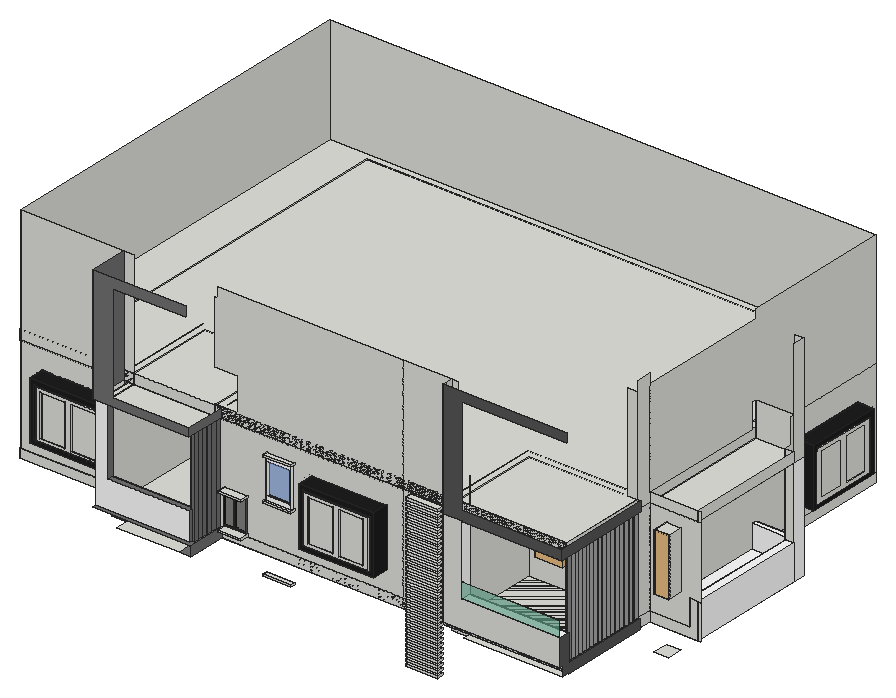
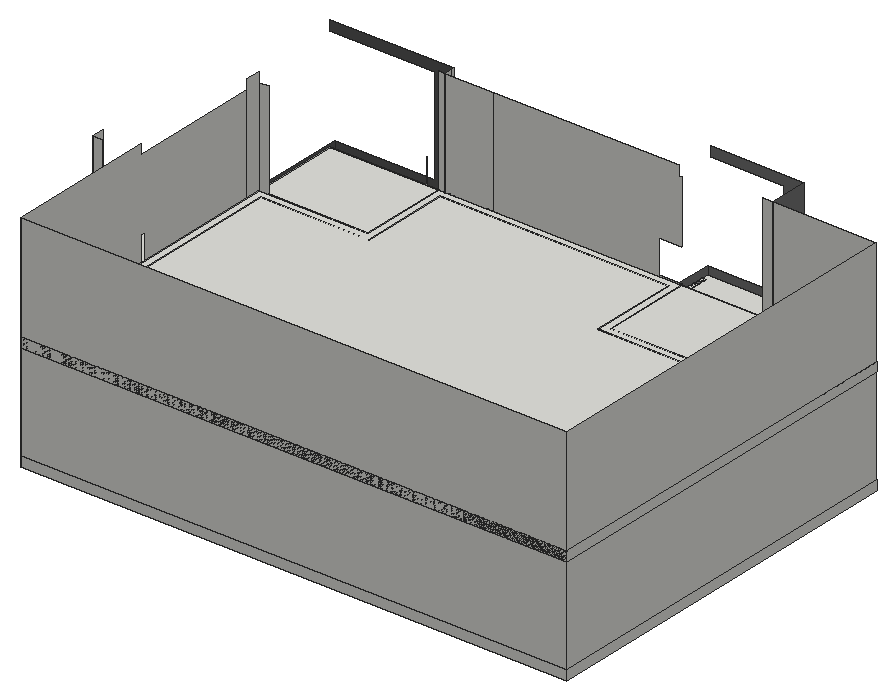
# SketchUp Ruby script. Lengths in inches.
U = 1.inch
M = Sketchup.active_model
def pt(a) = Geom::Point3d.new(a.map { |v| v * U })
def face(e, loops, mat)
  f = e.add_face(loops[0].map { |a| pt(a) })
  loops[1..].each { |l| e.add_face(l.map { |a| pt(a) }).erase! }
  f.material = f.back_material = mat if mat
  f
end
# faces: each face lists its corners as indices into pts; further lists are holes
def faces(e, pts, list, mat = nil) = list.each { |f| face(e, (f[0].is_a?(Array) ? f : [f]).map { |l| l.map { |i| pts[i] } }, mat) }
# xy, xz, yz: faces in a plane at the given z, y or x. An outline is a flat list of corners, or four numbers for a rectangle; further outlines are holes
def ring(l) = l.size == 4 ? [[l[0], l[1]], [l[2], l[1]], [l[2], l[3]], [l[0], l[3]]] : l.each_slice(2).to_a
def flat(e, list, mat, &to3) = list.each { |f| face(e, (f[0].is_a?(Array) ? f : [f]).map { |l| ring(l).map { |u, v| to3.(u, v) } }, mat) }
def xy(e, z, list, mat = nil) = flat(e, list, mat) { |x, y| [x, y, z] }
def xz(e, y, list, mat = nil) = flat(e, list, mat) { |x, z| [x, y, z] }
def yz(e, x, list, mat = nil) = flat(e, list, mat) { |y, z| [x, y, z] }
def lines(e, pts, list) = list.each { |a, b| e.add_line(pt(pts[a]), pt(pts[b])) }
# prism: a flat outline (further loops are holes) pulled along v
def prism(e, loops, v, mat = nil)
  f = face(e, loops, mat); d = Geom::Vector3d.new(v.map { |x| x * U })
  f.pushpull(f.normal.samedirection?(d) ? d.length : -d.length)
end
def box(e, o, s, mat = nil) = prism(e, [[o, [o[0] + s[0], o[1], o[2]], [o[0] + s[0], o[1] + s[1], o[2]], [o[0], o[1] + s[1], o[2]]]], [0, 0, s[2]], mat)
def at(x, y, z, deg = 0) = Geom::Transformation.translation(pt([x, y, z])) * Geom::Transformation.rotation(ORIGIN, Z_AXIS, deg.degrees)
def axes(o, x, y, z) = Geom::Transformation.new([*x, 0, *y, 0, *z, 0, *pt(o).to_a, 1])
def part(name) = M.definitions.add(name)
# library, detail: a bought-in or finely detailed component or shape, given as its bounding box
def library(name, o, s) = part(name).tap { |d| box(d.entities, o, s) }
def detail(e, o, s) = box(e.add_group.entities, o, s)
def put(e, d, t, mat = nil) = e.add_instance(d, t).tap { |i| i.material = mat if mat }
def group(e, t, mat = nil) = e.add_group.tap { |g| g.transformation = t; g.material = mat if mat }.entities
root = M.entities
M.materials.add("Glass_Tinted_Gray").color = [0, 0, 0]
M.materials["Glass_Tinted_Gray"].alpha = 0.125
M.materials.add("MaterialE").color = [182, 131, 172]
M.materials["MaterialE"].alpha = 0.66
M.materials.add("MaterialF").color = [114, 188, 161]
M.materials["MaterialF"].alpha = 0.66
M.materials.add("[0135_DarkGray]").color = [81, 81, 81]
M.materials.add("[Color M00]").color = [255, 255, 255]
M.materials.add("[Color M03]").color = [170, 170, 170]
M.materials.add("[Color M04]").color = [142, 142, 142]
M.materials.add("[Color M05]").color = [114, 114, 114]
M.materials.add("[Color M06]").color = [86, 86, 86]
M.materials.add("[Color M08]").color = [30, 30, 30]
M.materials.add("[Color_000]").color = [255, 255, 255]
M.materials.add("[Mirror 02]1").color = [229, 229, 229]
M.materials.add("[Terrazzo Light Blue]").color = [196, 214, 227]
M.materials.add("[Translucent Glass Blue]").color = [100, 149, 237]
M.materials["[Translucent Glass Blue]"].alpha = 0.5
c1 = part("Group\#4")
box(c1.entities,[0,0,0],[39.5625,8.625,2.78])
c2 = part("Group\#73")
box(c2.entities,[0,0,0],[34.1875,2.25,6.125])
c3 = part("Group\#3")
box(c3.entities,[3,0,0],[2.8125,4.1875,120.875])
c4 = part("Group\#76")
box(c4.entities,[0,0,0],[4.8125,4.8125,120],"[Color M05]")
c5 = part("Group\#75")
box(c5.entities,[0,-10.375,0],[28.375,10.375,2.5])
c6 = part("PENTEK_RP Fineline 50S_Sliding_DoorCase_E1")
box(c6.entities,[0,0,0],[1.51,3.66,99.27],"[0135_DarkGray]")
c7 = part("PENTEK_RP Fineline 50S_SlidingDooe_Case_E2")
box(c7.entities,[0,0,0],[96.25,3.66,1.51],"[0135_DarkGray]")
c8 = part("pentek_RP Fineline 50S_SlidingDoor_Case")
put(c8.entities,c6,at(97.76,0,0))
put(c8.entities,c7,at(1.51,0,0))
put(c8.entities,c6,at(0,0,0))
put(c8.entities,c7,at(1.51,0,97.76))
c9 = part("PENTEK_RP Fineline 50S_SlidingDoor_GlazingBead_2")
box(c9.entities,[0,0,0],[0.56,0.59,94.39],"[0135_DarkGray]")
c10 = part("PENTEK_RP Fineline 50S_SlidingDoor_Glass")
box(c10.entities,[0,0,0],[46.58,0.16,94.39],"Glass_Tinted_Gray")
c11 = part("PENTEK_RP Fineline 50S_SlidingDoor_GlazingBead")
box(c11.entities,[0,0,0],[45.47,0.59,0.56],"[0135_DarkGray]")
c12 = part("PENTEK_RP Fineline 50S_SlidingDoor_Leaf_E1")
xy(c12.entities,0,[[0,0,0.93,1.97],[0.93,1.57,1.49,1.97]],"[0135_DarkGray]")
xy(c12.entities,96.25,[[0,0,0.93,0,0.93,1.57,1.49,1.57,1.49,1.97,0,1.97]],"[0135_DarkGray]")
xz(c12.entities,0,[[0,0,0.93,96.25]],"[0135_DarkGray]")
xz(c12.entities,1.57,[[0.93,0,1.49,95.32],[0.93,95.32,1.49,96.25]],"[0135_DarkGray]")
xz(c12.entities,1.97,[[0,0,1.49,96.25]],"[0135_DarkGray]")
yz(c12.entities,0,[[0,0,1.97,96.25]],"[0135_DarkGray]")
yz(c12.entities,0.93,[[0,0,1.57,0.93],[0,0.93,1.57,95.32],[0,95.32,1.57,96.25]],"[0135_DarkGray]")
yz(c12.entities,1.49,[[1.57,0,1.97,95.32],[1.57,95.32,1.97,96.25]],"[0135_DarkGray]")
c13 = part("PENTEK_RP Fineline 50S_SlidingDoor_Leaf_E2")
xy(c13.entities,0,[[0,0,0,1.57,0.56,1.57,0.56,1.97,46.02,1.97,46.02,1.57,46.58,1.57,46.58,0]],"[0135_DarkGray]")
xy(c13.entities,0.93,[[0,0,46.58,1.57]],"[0135_DarkGray]")
xy(c13.entities,1.49,[[0.56,1.57,46.02,1.97]],"[0135_DarkGray]")
xz(c13.entities,0,[[0,0,46.58,0.93]],"[0135_DarkGray]")
xz(c13.entities,1.57,[[0,0,0.56,0.93],[46.02,0,46.58,0.93],[0.56,0.93,46.02,1.49]],"[0135_DarkGray]")
xz(c13.entities,1.97,[[0.56,0,46.02,1.49]],"[0135_DarkGray]")
yz(c13.entities,0,[[0,0,1.57,0.93]],"[0135_DarkGray]")
yz(c13.entities,0.56,[[1.57,0,1.97,0.93],[1.57,0.93,1.97,1.49]],"[0135_DarkGray]")
yz(c13.entities,46.02,[[1.57,0,1.97,0.93],[1.57,0.93,1.97,1.49]],"[0135_DarkGray]")
yz(c13.entities,46.58,[[0,0,1.57,0.93]],"[0135_DarkGray]")
c14 = part("PENTEK_RP Fineline S_SlidingDoor_Leaf1")
put(c14.entities,c9,at(0.93,0,0.93))
put(c14.entities,c9,at(46.96,0,0.93))
put(c14.entities,c10,at(1.49,1.42,0.93))
put(c14.entities,c11,at(1.49,0,0.93))
put(c14.entities,c10,at(1.49,0.59,0.93),"[Terrazzo Light Blue]")
put(c14.entities,c12,at(0,0,0))
put(c14.entities,c12,axes([48.44,0,0],[-1,0,0],[0,1,0],[0,0,1]))
put(c14.entities,c13,axes([0.93,0,96.25],[1,0,0],[0,1,0],[0,0,-1]))
put(c14.entities,c13,at(0.93,0,0))
put(c14.entities,c11,at(1.49,0,94.77))
c15 = part("PENTEK_RP Fineline 50S_SlidingDoor_Leaf2")
put(c15.entities,c10,at(1.49,1.42,0.93))
put(c15.entities,c11,at(1.49,0,94.77))
put(c15.entities,c9,at(46.96,0,0.93))
put(c15.entities,c10,at(1.49,0.59,0.93),"[Mirror 02]1")
put(c15.entities,c9,at(0.93,0,0.93))
put(c15.entities,c12,at(0,0,0))
put(c15.entities,c12,axes([48.44,0,0],[-1,0,0],[0,1,0],[0,0,1]))
put(c15.entities,c11,at(1.49,0,0.93))
put(c15.entities,c13,axes([0.93,0,96.25],[1,0,0],[0,1,0],[0,0,-1]))
put(c15.entities,c13,at(0.93,0,0))
c16 = part("PENTEK - Slimmest Steel Sliding Door / Window\#1")
put(c16.entities,c8,at(0,-1.88,-0.09))
put(c16.entities,c14,at(1.51,-2.27,1.42))
put(c16.entities,c15,at(49.32,-0.3,1.42))
c17 = library("Single door",[0,0,0],[7.5,39.86,83.92])
c18 = part("Window")
xy(c18.entities,31.72,[[-0.78,88.6,2.72,128.1]])
xy(c18.entities,34.95,[[-0.78,91.53,0.84,106.59],[0.84,91.53,1.05,97.58],[1.05,91.53,1.42,106.59],[1.42,91.53,2.72,106.59],[0.84,97.58,1.05,98.18],
  [0.84,98.18,1.05,106.59]])
xy(c18.entities,35.27,[[-0.78,110.09,0.97,125.14],[1.05,110.09,2.72,125.14]])
xy(c18.entities,58.35,[[2.72,108.74,3.8,109.74]])
xy(c18.entities,77.8125,[[-0.78,110.09,2.72,125.14],[0.97,110.09,1.05,125.14]])
xy(c18.entities,77.93,[[-0.78,91.53,0.84,106.59],[1.05,91.53,1.42,106.59],[1.42,91.53,2.72,106.59]])
xy(c18.entities,80.72,[[-0.78,88.6,2.72,128.1]])
xz(c18.entities,88.6,[[-0.78,31.72,2.72,80.72]])
xz(c18.entities,91.53,[[-0.78,34.95,0.84,77.93],[1.05,34.95,1.42,77.93],[1.42,34.95,2.72,77.93]])
xz(c18.entities,106.59,[[-0.78,34.95,0.84,77.93],[0.84,34.95,1.05,77.93],[0.84,34.95,2.72,77.93]])
xz(c18.entities,108.74,[[3.8,54.35,4.22,54.6,4.22,59.47,2.72,59.97,2.72,58.35,3.8,58.35]])
xz(c18.entities,109.74,[[3.8,54.35,3.8,58.35,2.72,58.35,2.72,59.97,4.22,59.47,4.22,54.6]])
xz(c18.entities,110.09,[[-0.78,35.27,0.97,77.8125],[1.05,35.27,2.72,77.8125]])
xz(c18.entities,125.14,[[-0.78,35.27,0.97,77.8125],[0.97,35.27,1.05,80.72],[1.05,35.27,2.72,77.8125]])
xz(c18.entities,128.1,[[-0.78,31.72,2.72,80.72]])
yz(c18.entities,-0.78,[[[88.6,31.72,128.1,80.72],[91.53,34.95,106.59,77.93],[110.09,35.27,125.14,77.8125]]])
yz(c18.entities,0.84,[[91.53,34.95,106.59,77.93]])
yz(c18.entities,0.97,[[110.09,35.27,125.14,77.8125]])
yz(c18.entities,1.05,[[91.53,34.95,106.59,77.93],[110.09,35.27,125.14,77.8125]])
yz(c18.entities,1.42,[[91.53,34.95,106.59,77.93]])
yz(c18.entities,2.72,[[[88.6,31.72,108.35,80.72],[91.53,34.95,106.59,77.93]],[[108.35,31.72,128.1,80.72],[110.09,35.27,125.14,77.8125],[108.74,58.35,109.74,59.97]]])
yz(c18.entities,3.8,[[108.74,54.35,109.74,58.35]])
yz(c18.entities,4.22,[[108.74,54.6,109.74,59.47]])
p = [[4.22,108.74,54.6],[3.8,108.74,54.35],[3.8,109.74,54.35],[4.22,109.74,54.6],[2.72,109.74,59.97],[2.72,108.74,59.97],
  [4.22,108.74,59.47],[4.22,109.74,59.47],[-0.78,86.4,89.94],[-0.78,86.44,89.94],[15.22,130.69,89.94],[15.22,130.65,89.94],
  [-0.78,86.44,28.19],[-0.78,86.4,28.19],[7.72,130.69,89.94],[7.72,130.65,89.94]]
faces(c18.entities,p,[[0,1,2,3],[4,5,6,7]])
lines(c18.entities,p,[[8,9],[10,11],[12,13],[14,15]])
c19 = part("Group\#5")
xy(c19.entities,0,[[[0,0,93.5,72.0625],[5.4,5.4,88.1,66.66]],[5.4,5.4,88.1,66.66]])
xy(c19.entities,20.1875,[[[0,0,93.5,72.0625],[5.4,5.4,88.1,66.66]]])
xz(c19.entities,0,[[0,0,93.5,20.1875]])
xz(c19.entities,5.4,[[5.4,0,88.1,20.1875]])
xz(c19.entities,66.66,[[5.4,0,88.1,20.1875]])
xz(c19.entities,72.0625,[[0,0,93.5,20.1875]])
yz(c19.entities,0,[[0,0,72.0625,20.1875]])
yz(c19.entities,5.4,[[5.4,0,66.66,20.1875]])
yz(c19.entities,88.1,[[5.4,0,66.66,20.1875]])
yz(c19.entities,93.5,[[0,0,72.0625,20.1875]])
c20 = library("Sliding Window",[0,0,0],[35.43,4.93,59.06])
c21 = part("glassE")
xy(c21.entities,0,[[0,0,37.99,0.79]],"MaterialE")
xy(c21.entities,38.27,[[0,0,37.99,0.79]],"MaterialE")
xz(c21.entities,0,[[0,0,37.99,38.27]],"MaterialF")
yz(c21.entities,0,[[0,0,0.79,38.27]],"MaterialE")
yz(c21.entities,37.99,[[0,0,0.79,38.27]],"MaterialE")
c22 = library("grille P1",[0,0,0],[0.79,28.9,72.83])
c23 = part("bod vindu")
g1 = group(c23.entities,at(0,-46.85,0),"[Translucent Glass Blue]")
yz(g1,0.94,[[2.36,2.36,44.49,19.65]],"[Translucent Glass Blue]")
p = [[0.55,44.49,2.36],[0.94,44.49,2.36],[0.55,2.36,19.65],[0.94,2.36,19.65]]
lines(g1,p,[[0,1],[2,3]])
g2 = group(g1,at(0,46.85,0,-90),"[Color_000]")
xy(g2,0,[[0,0,46.85,3.9375]])
xy(g2,1.57,[[1.57,0,45.28,0.55]])
xy(g2,2.36,[[2.36,0.55,44.49,3.9375]])
xy(g2,19.65,[[2.36,0.55,4.29,3.9375],[4.29,0.55,44.49,3.9375]])
xy(g2,20.43,[[1.57,0,45.28,0.55]])
xy(g2,22.01,[[0,0,46.85,3.9375]])
xz(g2,0,[[[0,0,46.85,22.01],[1.57,1.57,45.28,20.43]]])
xz(g2,0.55,[[1.57,1.57,45.28,2.36],[1.57,2.36,2.36,2.36,2.36,19.65,44.49,19.65,44.49,2.36,45.28,2.36,45.28,20.43,1.57,20.43]])
xz(g2,3.9375,[[[0,0,46.85,22.01],[2.36,2.36,44.49,19.65]]])
yz(g2,0,[[0,0,3.9375,22.01]])
yz(g2,1.57,[[0,1.57,0.55,2.36,0.55,20.43,0,20.43]])
yz(g2,2.36,[[0.55,2.36,3.9375,19.65]])
yz(g2,44.49,[[0.55,2.36,3.9375,19.65]])
yz(g2,45.28,[[0,1.57,0,20.43,0.55,20.43,0.55,2.36]])
yz(g2,46.85,[[0,0,3.9375,22.01]])
p = [[45.28,0,1.57],[1.57,0,1.57],[1.57,0.55,2.36],[2.36,0.55,2.36],[44.49,0.55,2.36],[45.28,0.55,2.36]]
faces(g2,p,[[0,1,2,3,4,5]])
xy(root,233.98,[[848.78,313.75,867.09,332.62]])
xy(root,252,[[308.96,155.5,308.96,170.3125,291.14,170.3125,291.14,203.9375,386.69,203.9375,386.69,155.5],[386.69,170.3125,392.02,203.9375],[[150.47,203.9375,291.32,203.9375,291.32,313.75,392.02,313.75,392.02,203.9375,693.39,203.9375,693.39,313.75,827.97,313.75,827.97,683.9375,150.47,683.9375],[203.47,212.9375,203.47,674.9375,818.97,674.9375,818.97,322.75,684.39,322.75,684.39,212.9375,401.02,212.9375,401.02,322.75,282.32,322.75,282.32,212.9375]],[818.5,203.9375,827.97,313.75],[828.01,203.9375,830.59,313.75]])
xy(root,252,[[827.97,332.62,887.97,496.51]],"[Color M00]")
xy(root,252,[[386.69,155.5,400.83,170.3125],[392.02,170.3125,400.83,203.9375]],"[Color M05]")
xy(root,252.02,[[707.95,194.4375,830.59,203.9375]])
xy(root,264,[[[284.94,166.84,291.32,166.84,291.32,313.75,392.02,313.75,392.02,203.9375,693.39,203.9375,693.39,313.75,827.97,313.75,827.97,683.9375,150.47,683.9375,150.47,203.9375,284.94,203.9375],[203.47,212.9375,203.47,674.9375,818.97,674.9375,818.97,322.75,684.39,322.75,684.39,212.9375,401.02,212.9375,401.02,322.75,282.32,322.75,282.32,212.9375]],[685.61,190.6875,830.59,194.4375],[685.61,194.4375,830.59,203.9375],[693.39,203.9375,827.97,313.75],[203.47,212.9375,282.32,212.9375,282.32,322.75,401.02,322.75,401.02,212.9375,684.39,212.9375,684.39,322.75,818.97,322.75,818.97,674.9375,203.47,674.9375]])
xy(root,264,[[827.97,332.62,827.97,490.24,876.25,490.24,876.25,481.58,877.14,481.58,877.14,332.62]],"[Color M00]")
xy(root,264,[[278.57,155.5,400.83,155.5,400.83,203.9375,392.02,203.9375,392.02,313.75,291.32,313.75,291.32,166.84,395.25,166.84,395.25,160.4375,278.57,160.4375]],"[Color M05]")
xy(root,264,[[828.01,203.9375,830.59,313.75]],"[Color M06]")
xy(root,292.1875,[[827.97,490.24,876.25,496.51]],"[Color M00]")
xy(root,295.27,[[877.14,332.62,887.97,481.58]],"[Color M00]")
xy(root,297,[[707.95,190.6875,830.59,203.9375]],"[Color M00]")
xy(root,298.79,[[848.78,313.75,867.09,332.62]])
xy(root,299.125,[[294.36,160.4375,395.25,166.84]],"[Color M05]")
xy(root,369.91,[[848.78,313.75,867.09,332.62]])
xy(root,384,[[278.57,155.5,278.57,160.4375,294.36,160.4375,294.36,166.84,291.32,166.84,291.32,203.9375,398.77,203.9375,398.77,155.5],[284.94,166.84,291.32,203.9375],[685.61,190.6875,707.95,203.9375],[707.95,190.6875,707.95,203.9375,827.97,203.9375,827.97,313.75,832.47,313.75,832.47,190.6875],[150.47,203.9375,150.47,683.9375,827.97,683.9375,827.97,313.75,693.39,313.75,693.39,203.9375,392.02,203.9375,392.02,313.75,291.32,313.75,291.32,203.9375],
  [827.97,332.62,887.97,496.51]])
xz(root,155.5,[[278.57,384,398.77,384,398.77,394.01,304.51,394.01,304.51,516,395.02,516,395.02,528,278.57,528]],"[Color M05]")
xz(root,160.4375,[[278.57,264,395.25,264,395.25,299.125,294.36,299.125,294.36,384,278.57,384]],"[Color M00]")
xz(root,166.84,[[291.32,264,291.32,384,294.36,384,294.36,299.125,395.25,299.125,395.25,264]],"[Color M05]")
xz(root,190.6875,[[685.61,264,830.59,264,830.59,297,707.95,297,707.95,384,685.61,384]])
xz(root,190.6875,[[685.61,384,832.47,384,832.47,396,707.95,396,707.95,516,838.2,516,838.2,528,685.61,528]],"[Color M06]")
xz(root,203.9375,[[685.61,249.15,693.39,252],[693.39,249.15,707.95,252],[400.83,252,624.38,264],[624.38,252,685.61,264],[685.61,252,685.61,264,828.01,264,828.01,252.02,707.95,252.02,707.95,252],
  [828.01,252,830.59,252.02],[150.47,264,278.57,384],[392.02,264,624.38,384],[624.38,264,685.61,384],[685.61,264,693.39,384],
  [693.39,264,787.85,264,787.85,297,707.95,297,707.95,277.375,693.39,277.375],[787.85,264,827.97,297],[827.97,264,828.01,297],[828.01,264,830.59,297],[693.39,277.375,707.95,384],
  [150.47,384,278.57,528],[278.57,384,291.32,528],[392.02,384,398.77,394.01],[398.77,384,624.38,384,624.38,528,395.02,528,395.02,516,392.02,516,392.02,438.17,420.4,438.17,420.4,397.79,392.02,397.79,392.02,394.01,398.77,394.01],[624.38,384,685.61,528],
  [685.61,384,693.39,528],[693.39,384,693.39,396,707.82,396,707.82,428,707.95,428,707.95,396,827.97,396,827.97,384]])
xz(root,203.9375,[[278.57,264,284.94,384]],"[Color M05]")
xz(root,212.9375,[[203.47,264,282.32,384],[401.02,264,684.39,384],[203.47,384,282.32,396],[401.02,384,684.39,396]])
xz(root,313.75,[[828.01,252,830.59,264],[291.32,264,392.02,384],[693.39,264,827.97,384],[291.32,384,392.02,396],[693.39,384,816.38,396],
  [816.38,384,827.97,516],[827.97,384,832.47,396]])
xz(root,322.75,[[282.32,264,401.02,384],[684.39,264,818.97,384],[282.32,384,401.02,396],[684.39,384,818.97,396]])
xz(root,332.62,[[827.97,252,827.97,264,877.14,264,877.14,295.27,887.97,295.27,887.97,252],[887.97,252,891.78,295.27],[[827.97,264,827.97,384,891.78,384,891.78,295.27,877.14,295.27,877.14,264],[848.78,298.79,867.09,369.91]],[827.97,384,887.97,396],[887.97,384,891.78,396]])
xz(root,481.58,[[876.25,264,877.14,264,877.14,295.27,887.97,295.27,887.97,396,876.25,396]])
xz(root,490.24,[[827.97,264,876.25,292.1875]],"[Color M00]")
xz(root,496.51,[[827.97,384,876.25,426.875],[876.25,384,887.97,516]])
xz(root,496.51,[[827.97,252,876.25,292.1875],[876.25,252,887.97,384]],"[Color M00]")
xz(root,674.9375,[[203.47,264,818.97,384],[203.47,384,818.97,396]])
xz(root,683.9375,[[150.47,264,827.97,384],[150.47,384,827.97,528]])
yz(root,150.47,[[203.9375,264,683.9375,384],[203.9375,384,683.9375,528]])
yz(root,203.47,[[212.9375,264,674.9375,384],[212.9375,384,674.9375,396]])
yz(root,278.57,[[155.5,384,203.9375,528]],"[Color M05]")
yz(root,282.32,[[212.9375,264,322.75,384],[212.9375,384,322.75,396]])
yz(root,284.94,[[166.84,264,203.9375,384]],"[Color M05]")
yz(root,291.32,[[166.84,264,313.75,384],[203.9375,384,313.75,396]])
yz(root,294.36,[[160.4375,299.125,166.84,384]],"[Color M05]")
yz(root,392.02,[[203.9375,264,313.75,384],[203.9375,384,313.75,396]])
yz(root,395.25,[[160.4375,264,166.84,299.125]],"[Color M05]")
yz(root,398.77,[[155.5,384,203.9375,394.01]],"[Color M05]")
yz(root,400.83,[[155.5,252,203.9375,264]],"[Color M05]")
yz(root,401.02,[[212.9375,264,322.75,384],[212.9375,384,322.75,396]])
yz(root,684.39,[[212.9375,264,322.75,384],[212.9375,384,322.75,396]])
yz(root,685.61,[[190.6875,264,194.4375,384],[194.4375,264,203.9375,384],[190.6875,384,194.4375,528],[194.4375,384,203.9375,528]])
yz(root,693.39,[[203.9375,264,313.75,384],[203.9375,384,313.75,396]])
yz(root,707.95,[[190.6875,297,203.9375,384]],"[Color M00]")
yz(root,818.97,[[322.75,264,674.9375,384],[322.75,384,674.9375,396]])
yz(root,827.97,[[313.75,252,332.62,264],[313.75,264,332.62,384],[332.62,264,490.24,264,490.24,292.1875,496.51,292.1875,496.51,264,683.9375,264,683.9375,384,332.62,384],[203.9375,384,313.75,396],[313.75,384,332.62,528],
  [496.51,384,683.9375,384,683.9375,528,496.51,528,496.51,516,332.62,516,332.62,396,490.94,396,490.94,426.875,496.51,426.875]])
yz(root,827.97,[[490.24,264,496.51,292.1875]],"[Color M00]")
yz(root,828.01,[[203.9375,252,313.75,264]])
yz(root,830.59,[[203.9375,252,313.75,252,313.75,264,203.9375,264,203.9375,297,190.6875,297,190.6875,264,194.4375,264,194.4375,252.02,203.9375,252.02]],"[Color M06]")
yz(root,832.47,[[190.6875,384,313.75,396]],"[Color M06]")
yz(root,848.78,[[313.75,298.79,332.62,369.91]])
yz(root,867.09,[[313.75,298.79,332.62,369.91]])
yz(root,876.25,[[481.58,264,481.58,396,490.94,396,490.94,426.875,496.51,426.875,496.51,292.1875,490.24,292.1875,490.24,264]])
yz(root,877.14,[[332.62,264,481.58,295.27]],"[Color M00]")
yz(root,887.97,[[332.62,384,481.58,396],[481.58,384,496.51,516]])
yz(root,887.97,[[332.62,252,481.58,295.27],[481.58,252,496.51,384]],"[Color M00]")
put(root,c1,at(635.73,194.4375,195.88))
put(root,c1,at(635.73,194.4375,201.45))
put(root,c1,at(635.73,194.4375,207.01))
put(root,c1,at(635.73,194.4375,212.57))
put(root,c1,at(635.73,194.4375,218.13))
put(root,c1,at(635.73,194.4375,223.7))
put(root,c1,at(635.73,194.4375,229.26))
put(root,c2,axes([456.17,203.9375,231.33],[1,0,0],[0,0,1],[0,-1,0]))
put(root,c1,at(635.73,194.4375,234.82))
put(root,c1,at(635.73,194.4375,240.38))
put(root,c1,at(635.73,194.4375,245.95))
put(root,c1,at(635.73,194.4375,251.51))
g3 = group(root,at(193.09,683.9375,252))
box(g3,[-42.625,-480,0],[677.5,480,12])
put(root,c1,at(635.73,194.4375,257.07))
put(root,c1,at(635.73,194.4375,262.63))
put(root,c3,at(822.2,206.09,264),"[Color M04]")
put(root,c3,at(822.2,211.97,264),"[Color M03]")
put(root,c3,at(822.2,217.53,264),"[Color M03]")
put(root,c3,at(822.2,223.03,264),"[Color M03]")
put(root,c3,at(822.2,228.66,264),"[Color M03]")
put(root,c3,at(822.2,234.66,264),"[Color M03]")
put(root,c3,at(822.2,240.47,264),"[Color M03]")
put(root,c3,at(822.2,246.66,264),"[Color M03]")
put(root,c3,at(822.2,253.03,264),"[Color M03]")
put(root,c3,at(822.2,259.78,264),"[Color M03]")
put(root,c3,at(822.2,266.41,264),"[Color M03]")
put(root,c3,at(822.2,273.09,264),"[Color M03]")
put(root,c3,at(822.2,280.28,264),"[Color M03]")
put(root,c3,at(822.2,286.84,264),"[Color M03]")
put(root,c3,at(822.2,294.28,264),"[Color M03]")
put(root,c3,at(822.2,301.47,264),"[Color M03]")
put(root,c3,at(822.2,309.59,264),"[Color M03]")
put(root,c4,at(393.9,197.98,264))
put(root,c4,at(393.9,191.1,264))
put(root,c4,at(393.9,183.91,264))
put(root,c4,at(393.9,177.04,264))
put(root,c4,at(393.9,170.66,264))
put(root,c4,at(393.9,163.79,264))
put(root,c5,at(403.93,203.9375,264.08))
put(root,c16,axes([403.24,203.32,267.14],[0.27919,0,0],[0,0.34311,0],[0,0,0.40008]))
put(root,c17,at(760.44,316.08,267.3125,-90))
put(root,c1,at(635.73,194.4375,268.2))
put(root,c1,at(635.73,194.4375,273.76))
put(root,c1,at(635.73,194.4375,279.32))
put(root,c1,at(635.73,194.4375,284.88))
put(root,c18,axes([852.91,821.1,252.45],[-1,0,0],[0,-2.03871,0],[0,0,1.22883]))
put(root,c19,axes([833.5,554.66,287.09],[0,1,0],[0,0,1],[1,0,0]),"[Color M08]")
put(root,c19,axes([177.81,203.9375,287.32],[1,0,0],[0,0,1],[0,-1,0]),"[Color M08]")
put(root,c18,axes([778.5,184.53,252.96],[0,1,0],[-2.03871,0,0],[0,0,1.22883]))
put(root,c18,axes([446.4375,184.53,252.96],[0,1,0],[-2.03871,0,0],[0,0,1.22883]))
put(root,c19,axes([512.06,203.9375,287.6],[1,0,0],[0,0,1],[0,-1,0]),"[Color M08]")
put(root,c1,at(635.73,194.4375,290.88))
put(root,c20,at(704.35,308.67,291.3125))
put(root,c1,at(635.73,194.4375,296.88))
put(root,c21,axes([707.95,190.6875,297],[3.2107,0,0],[0,1.17,0],[0,0,0.5016]))
put(root,c22,axes([867.09,313.75,298.54],[0,1,0],[-0.61577,0,0],[0,0,0.98]))
put(root,c1,at(635.73,194.4375,302.88))
put(root,c5,at(403.93,203.9375,306.96))
put(root,c1,at(635.73,194.4375,308.88))
put(root,c2,axes([456.17,203.9375,312.74],[1,0,0],[0,0,1],[0,-1,0]))
put(root,c1,at(635.73,194.4375,314.88))
put(root,c23,axes([488.85,203.9375,314.99],[0,-1,0],[0.6656,0,0],[0,0,2.2308]))
put(root,c1,at(635.73,194.4375,320.88))
put(root,c1,at(635.73,194.4375,326.88))
put(root,c1,at(635.73,194.4375,332.88))
put(root,c1,at(635.73,194.4375,338.88))
put(root,c1,at(635.73,194.4375,344.88))
put(root,c1,at(635.73,194.4375,350.88))
put(root,c1,at(635.73,194.4375,356.88))
put(root,c1,at(635.73,194.4375,362.88))
put(root,c2,axes([456.17,203.9375,364.08],[1,0,0],[0,0,1],[0,-1,0]))
put(root,c1,at(635.73,194.4375,368.88))
put(root,c1,at(635.73,194.4375,374.88))
put(root,c1,at(635.73,194.4375,380.88))
g4 = group(root,at(193.09,683.9375,384))
box(g4,[-42.625,-480,0],[677.5,480,12])
